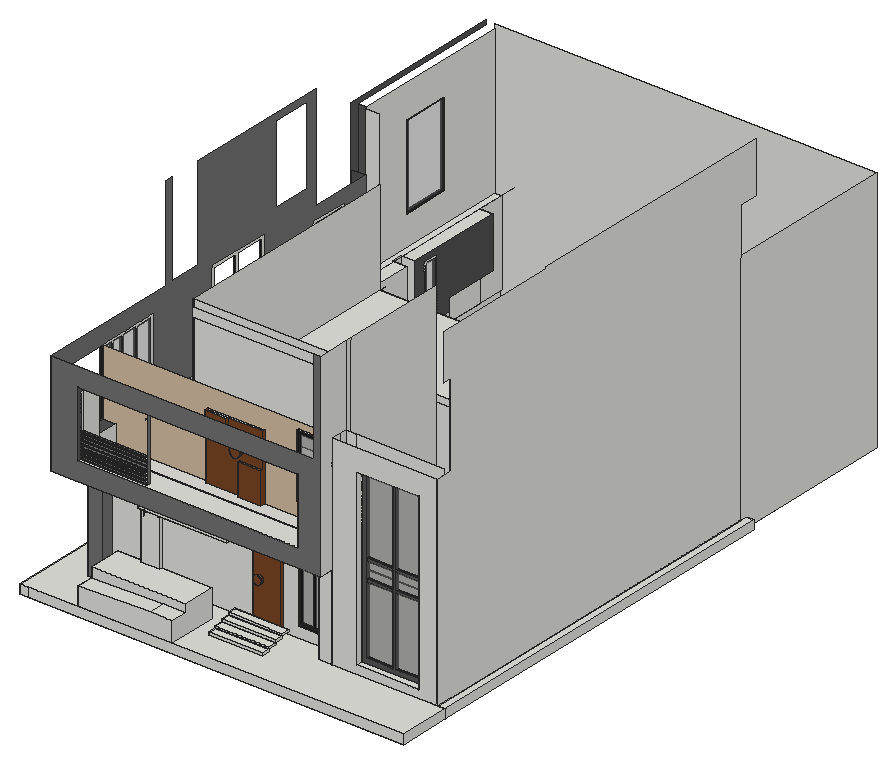
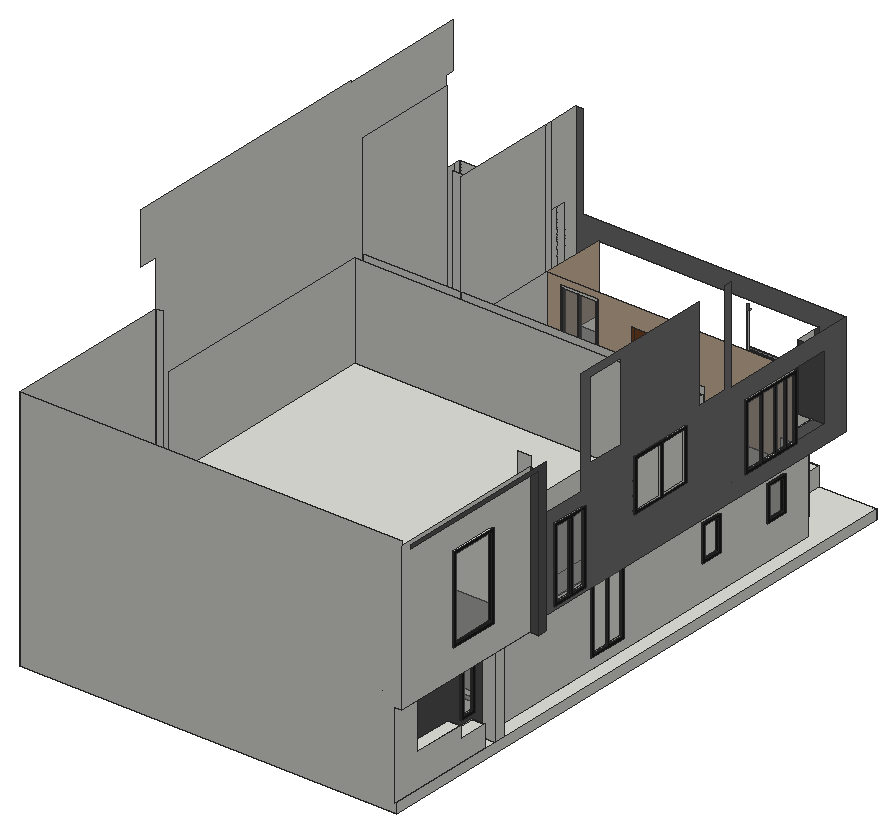
# SketchUp Ruby script. Lengths in inches.
U = 1.inch
M = Sketchup.active_model
def pt(a) = Geom::Point3d.new(a.map { |v| v * U })
def face(e, loops, mat)
  f = e.add_face(loops[0].map { |a| pt(a) })
  loops[1..].each { |l| e.add_face(l.map { |a| pt(a) }).erase! }
  f.material = f.back_material = mat if mat
  f
end
# faces: each face lists its corners as indices into pts; further lists are holes
def faces(e, pts, list, mat = nil) = list.each { |f| face(e, (f[0].is_a?(Array) ? f : [f]).map { |l| l.map { |i| pts[i] } }, mat) }
# xy, xz, yz: faces in a plane at the given z, y or x. An outline is a flat list of corners, or four numbers for a rectangle; further outlines are holes
def ring(l) = l.size == 4 ? [[l[0], l[1]], [l[2], l[1]], [l[2], l[3]], [l[0], l[3]]] : l.each_slice(2).to_a
def flat(e, list, mat, &to3) = list.each { |f| face(e, (f[0].is_a?(Array) ? f : [f]).map { |l| ring(l).map { |u, v| to3.(u, v) } }, mat) }
def xy(e, z, list, mat = nil) = flat(e, list, mat) { |x, y| [x, y, z] }
def xz(e, y, list, mat = nil) = flat(e, list, mat) { |x, z| [x, y, z] }
def yz(e, x, list, mat = nil) = flat(e, list, mat) { |y, z| [x, y, z] }
def lines(e, pts, list) = list.each { |a, b| e.add_line(pt(pts[a]), pt(pts[b])) }
# prism: a flat outline (further loops are holes) pulled along v
def prism(e, loops, v, mat = nil)
  f = face(e, loops, mat); d = Geom::Vector3d.new(v.map { |x| x * U })
  f.pushpull(f.normal.samedirection?(d) ? d.length : -d.length)
end
def box(e, o, s, mat = nil) = prism(e, [[o, [o[0] + s[0], o[1], o[2]], [o[0] + s[0], o[1] + s[1], o[2]], [o[0], o[1] + s[1], o[2]]]], [0, 0, s[2]], mat)
def at(x, y, z, deg = 0) = Geom::Transformation.translation(pt([x, y, z])) * Geom::Transformation.rotation(ORIGIN, Z_AXIS, deg.degrees)
def axes(o, x, y, z) = Geom::Transformation.new([*x, 0, *y, 0, *z, 0, *pt(o).to_a, 1])
def part(name) = M.definitions.add(name)
# library, detail: a bought-in or finely detailed component or shape, given as its bounding box
def library(name, o, s) = part(name).tap { |d| box(d.entities, o, s) }
def detail(e, o, s) = box(e.add_group.entities, o, s)
def put(e, d, t, mat = nil) = e.add_instance(d, t).tap { |i| i.material = mat if mat }
def group(e, t, mat = nil) = e.add_group.tap { |g| g.transformation = t; g.material = mat if mat }.entities
root = M.entities
M.materials.add("[0135_DarkGray]").color = [81, 81, 81]
M.materials.add("[Color M04]").color = [142, 142, 142]
M.materials.add("[Color M05]").color = [114, 114, 114]
M.materials.add("[Color M06]").color = [86, 86, 86]
M.materials.add("[Color M08]").color = [30, 30, 30]
M.materials.add("[Formica Laminate Light]").color = [213, 189, 164]
M.materials.add("[Marble Carrara Gold Floor Tile]").color = [225, 223, 217]
M.materials.add("[Translucent Glass Gray]").color = [128, 128, 128]
M.materials["[Translucent Glass Gray]"].alpha = 0.5
M.materials.add("[Wood Veneer 01]").color = [120, 70, 37]
xy(root,0,[[25.8125,0,25.8125,764.77,496.75,764.77,496.75,539.83,52.75,539.83,52.75,95.83,496.75,95.83,496.75,65.83,514.75,65.83,514.75,0],[496.75,65.83,503.64,77.83],[505.75,65.83,505.75,548.83,496.75,548.83,496.75,557.83,514.5625,557.83,514.5625,65.83],[503.64,65.83,505.75,74.83],[514.5625,65.83,514.75,557.83],
  [503.64,74.83,505.75,77.83],[503.64,74.83,505.75,86.83],[496.75,77.83,503.64,86.83],[503.64,77.83,505.75,86.83],[496.75,86.83,505.75,548.83],
  [52.75,95.83,496.75,539.83],[496.75,557.83,505.75,764.77]])
xy(root,12,[[[25.8125,0,99.13,0,99.13,63.3125,219.63,63.3125,219.63,0,514.75,0,514.75,65.83,354.09,65.83,354.09,86.83,291.2,86.83,291.2,83.83,255.2,83.83,255.2,86.83,43.75,86.83,43.75,593.74,25.8125,593.74],[68.26,54.08,88.33,68.45]],[371,65.83,496.75,65.83,496.75,548.83,43.75,548.83,43.75,86.83,371,86.83],[354.09,65.83,371,71.14],[496.75,65.83,505.75,548.83],[505.75,65.83,514.5625,557.83],
  [514.5625,65.83,514.75,557.83],[354.09,71.14,371,77.83],[354.09,77.83,371,86.83],[255.2,83.83,291.2,86.83],[496.75,548.83,505.75,557.83],
  [25.8125,607.3,43.75,607.3,43.75,622.4375,27.5,622.4375,27.5,764.77,25.8125,764.77],[27.5,622.4375,43.75,661.04],[27.5,661.04,28,730.625]])
xy(root,22.28,[[401.81,65.83,481.49,74.83],[401.81,74.83,481.49,77.83]])
xy(root,27.41,[[40.75,384.07,43.75,435.13]])
xy(root,27.74,[[313.68,83.83,351.43,86.83]])
xy(root,28.28,[[407.81,74.83,441.65,77.83],[445.14,74.83,475.49,77.83]],"[Color M06]")
xy(root,30.41,[[40.75,387.07,43.75,407.93],[40.75,409.6,43.75,432.13]],"[Color M08]")
xy(root,30.74,[[316.68,83.83,332.55,86.83],[333.49,83.83,348.43,86.83]],"[Color M08]")
xy(root,37.84,[[191.95,0,219.63,21.5625]])
xy(root,38.99,[[27.5,622.4375,43.75,661.04]])
xy(root,47.35,[[40.75,621.29,43.75,642.29]],"[Color M08]")
xy(root,48,[[99.13,21.5625,219.63,21.5625,219.63,63.3125,155.71,63.3125,155.71,59.3125,132.52,59.3125,132.52,63.3125,99.13,63.3125]])
xy(root,50.35,[[40.75,624.29,43.75,639.29]],"[Color M08]")
xy(root,54.51,[[27.5,661.04,28,730.625],[28,661.04,43.75,730.625]])
xy(root,57.8125,[[40.75,230.03,43.75,257.85]])
xy(root,57.8125,[[40.75,126.28,43.75,154.1]],"[Color M08]")
xy(root,60.8125,[[40.75,129.28,43.75,151.1],[40.75,233.03,43.75,254.85]],"[Color M08]")
xy(root,96,[[255.2,83.83,291.2,86.83]],"[Wood Veneer 01]")
xy(root,97.43,[[316.68,83.83,332.55,86.83],[333.49,83.83,348.43,86.83]],"[Color M08]")
xy(root,99.8125,[[40.75,129.28,43.75,151.1],[40.75,233.03,43.75,254.85]],"[Color M08]")
xy(root,100.43,[[313.68,83.83,351.43,86.83]],"[Color M08]")
xy(root,102.8125,[[40.75,126.28,43.75,154.1],[40.75,230.03,43.75,257.85]],"[Color M08]")
xy(root,108.125,[[132.52,59.3125,155.71,59.83],[127.97,59.83,132.52,63.3125],[155.71,59.83,155.71,63.3125,127.97,63.3125,127.97,86.83,241.41,86.83,241.41,59.83],[132.52,59.83,135.6,63.3125]])
xy(root,110.03,[[40.75,387.07,43.75,407.93],[40.75,409.6,43.75,432.13]])
xy(root,110.22,[[40.75,624.29,43.75,639.29]],"[Color M08]")
xy(root,113.03,[[40.75,384.07,43.75,435.13]],"[Color M08]")
xy(root,113.22,[[40.75,621.29,43.75,642.29]],"[Color M08]")
xy(root,115.77,[[407.81,74.83,441.65,77.83],[445.14,74.83,475.49,77.83]],"[Color M08]")
xy(root,118.37,[[407.81,74.83,441.65,77.83],[445.14,74.83,475.49,77.83]])
xy(root,120,[[354.09,65.83,371,71.14],[354.09,71.14,371,86.83],[342.51,95.83,371,230.47],[371,95.83,496.75,230.47],[51.5625,242.39,52.75,539.83],
  [52.75,242.39,496.75,539.83]])
xy(root,120,[[43.75,95.83,342.51,95.83,342.51,129.29,233.86,129.29,233.86,123.29,204.98,123.29,204.98,126.29,161.86,126.29,161.86,129.29,43.75,129.29]],"[Marble Carrara Gold Floor Tile]")
xy(root,120.1,[[19.75,548.83,19.75,764.77,27.5,764.77,27.5,730.625,43.75,730.625,43.75,607.3,25.8125,607.3,25.8125,593.74,43.75,593.74,43.75,548.83]])
xy(root,120.1,[[7.75,548.83,19.75,560.23]],"[Color M06]")
xy(root,120.125,[[27,47.14,27,548.83,43.75,548.83,43.75,86.83,127.97,86.83,127.97,59.83,241.41,59.83,241.41,86.83,371,86.83,371,47.14]])
xy(root,122.0625,[[371,85.64,496.75,86.83],[371,86.83,496.75,93.95],[371,93.95,496.75,95.83]])
xy(root,122.875,[[43.75,76.64,342.51,95.83]])
xy(root,127.17,[[24,465.2,27,514.14]],"[Color M08]")
xy(root,130.17,[[24,468.2,27,486.73],[24,489.67,27,511.14]],"[Color M08]")
xy(root,139.51,[[407.81,74.83,441.65,77.83],[445.14,74.83,475.49,77.83]],"[Color M08]")
xy(root,139.94,[[277.74,126.29,324.8,129.29]])
xy(root,140.6875,[[68.26,54.08,88.33,68.45]])
xy(root,142.35,[[407.81,74.83,441.65,77.83],[445.14,74.83,475.49,77.83]])
xy(root,142.94,[[280.74,126.29,301.27,129.29],[303.26,126.29,321.8,129.29]],"[Color M08]")
xy(root,144,[[146.02,47.14,342.51,47.14,342.51,76.64,61.54,76.64,61.54,55.45,146.02,55.45],[61.54,47.14,146.02,53.64],[61.54,53.64,145.89,55.45],[145.89,53.64,146.02,55.45],[43.75,76.64,61.54,80.27]])
xy(root,144,[[27,80.27,43.75,129.29]],"[0135_DarkGray]")
xy(root,144,[[24,129.29,27,209.85]],"[Color M08]")
xy(root,145.3125,[[61.54,49.95,146.02,53.64]])
xy(root,146.39,[[61.54,49.95,146.02,53.64]],"[Color M05]")
xy(root,147,[[24,132.29,27,144.3],[24,146.33,27,160.37],[24,161.62,27,182.61],[24,184.3,27,206.85]])
xy(root,149.6875,[[61.54,49.95,146.02,53.64]],"[Color M05]")
xy(root,150.77,[[61.54,49.95,146.02,53.64]],"[Color M05]")
xy(root,154.0625,[[61.54,49.95,146.02,53.64]],"[Color M05]")
xy(root,155.14,[[61.54,49.95,146.02,53.64]],"[Color M05]")
xy(root,157.5,[[16.75,621.57,19.75,684.82]],"[Color M08]")
xy(root,158.4375,[[61.54,49.95,146.02,53.64]],"[Color M05]")
xy(root,159.52,[[61.54,49.95,146.02,53.64]],"[Color M05]")
xy(root,160.11,[[204.98,123.29,233.86,126.29]],"[Wood Veneer 01]")
xy(root,160.5,[[16.75,624.57,19.75,681.82]],"[Color M08]")
xy(root,162.8125,[[61.54,49.95,146.02,53.64]],"[Color M05]")
xy(root,163.89,[[61.54,49.95,146.02,53.64]],"[Color M05]")
xy(root,167.1875,[[61.54,49.95,146.02,53.64]],"[Color M05]")
xy(root,168.27,[[61.54,49.95,146.02,53.64]],"[Color M05]")
xy(root,171.5625,[[61.54,49.95,146.02,53.64]],"[Color M05]")
xy(root,172.64,[[61.54,49.95,146.02,53.64]],"[Color M05]")
xy(root,175.66,[[24,303.96,27,386.64]],"[Color M08]")
xy(root,175.9375,[[61.54,49.95,146.02,53.64]],"[Color M05]")
xy(root,176.1875,[[161.86,123.29,189.67,126.29]],"[Wood Veneer 01]")
xy(root,177.02,[[61.54,49.95,146.02,53.64]],"[Color M05]")
xz(root,0,[[25.8125,0,34.75,12],[34.75,0,514.75,12],[99.13,12,219.63,12,219.63,37.84,191.95,37.84,99.13,35.36]])
xz(root,21.5625,[[99.13,35.36,191.95,37.84,219.63,37.84,219.63,48,99.13,48]])
xz(root,47.14,[[[27,120.125,371,120.125,371,372,362,372,362,252,27,252],[61.54,144,342.51,228.48]]],"[Color M05]")
xz(root,49.95,[[61.54,154.0625,146.02,155.14]],"[Color M04]")
xz(root,49.95,[[61.54,145.3125,146.02,146.39],[61.54,149.6875,146.02,150.77],[61.54,158.4375,146.02,159.52],[61.54,162.8125,146.02,163.89],[61.54,167.1875,146.02,168.27],
  [61.54,171.5625,146.02,172.64],[61.54,175.9375,146.02,177.02]],"[Color M05]")
xz(root,53.64,[[61.54,137.64,146.02,140.9375],[61.54,142.02,146.02,144],[145.89,144,146.02,145.3125],[61.54,145.3125,145.89,146.39],[145.89,145.3125,146.02,146.39],
  [145.89,146.39,146.02,149.6875],[61.54,149.6875,145.89,150.77],[145.89,149.6875,146.02,150.77],[145.89,150.77,146.02,154.0625],[61.54,154.0625,145.89,155.14],
  [145.89,154.0625,146.02,155.14],[145.89,155.14,146.02,158.4375],[61.54,158.4375,145.89,159.52],[145.89,158.4375,146.02,159.52],[145.89,159.52,146.02,162.8125],
  [61.54,162.8125,145.89,163.89],[145.89,162.8125,146.02,163.89],[145.89,163.89,146.02,167.1875],[61.54,167.1875,145.89,168.27],[145.89,167.1875,146.02,168.27],
  [145.89,168.27,146.02,171.5625],[61.54,171.5625,145.89,172.64],[145.89,171.5625,146.02,172.64],[145.89,172.64,146.02,175.9375],[61.54,175.9375,145.89,177.02],
  [145.89,175.9375,146.02,177.02],[145.89,177.02,146.02,180.3125]])
xz(root,54.08,[[68.26,12,88.33,140.6875]],"[Color M05]")
xz(root,55.45,[[145.89,144,146.02,220.77]])
xz(root,59.3125,[[132.52,48,155.71,108.125]])
xz(root,59.83,[[127.97,108.125,241.41,120.125]])
xz(root,63.3125,[[99.13,12,99.13,48,132.52,48,132.52,108.125,135.6,108.125,135.6,101.9375,155.71,101.9375,155.71,48,219.63,48,219.63,12],[135.6,101.9375,155.71,108.125]])
xz(root,65.83,[[496.75,0,503.64,12],[503.64,0,505.75,12],[505.75,0,514.5625,12],[514.5625,0,514.75,12],[354.09,12,371,120],
  [[371,12,503.64,270.8125],[401.81,22.28,481.49,243.28]],[503.64,12,505.75,270.8125]])
xz(root,68.45,[[68.26,12,88.33,140.6875]])
xz(root,71.14,[[354.09,12,371,120]])
xz(root,74.83,[[[401.81,22.28,481.49,243.28],[407.81,28.28,407.81,237.28,441.65,237.28,441.65,142.35,407.81,142.35,407.81,139.51,441.65,139.51,441.65,118.37,407.81,118.37,407.81,115.77,441.65,115.77,441.65,28.28],[445.14,142.35,475.49,237.28],[445.14,28.28,475.49,115.77],[445.14,118.37,475.49,139.51]]],"[Color M06]")
xz(root,76.64,[[43.75,122.875,342.51,144]])
xz(root,77.83,[[[401.81,22.28,481.49,243.28],[407.81,28.28,441.65,28.28,441.65,115.77,407.81,115.77,407.81,118.37,441.65,118.37,441.65,139.51,407.81,139.51,407.81,142.35,441.65,142.35,441.65,237.28,407.81,237.28],[445.14,142.35,475.49,237.28],[445.14,28.28,475.49,115.77],[445.14,118.37,475.49,139.51]]])
xz(root,77.83,[[407.81,28.28,441.65,115.77],[445.14,28.28,475.49,115.77],[407.81,118.37,441.65,139.51],[445.14,118.37,475.49,139.51],[407.81,142.35,441.65,237.28],
  [445.14,142.35,475.49,237.28]],"[Translucent Glass Gray]")
xz(root,80.27,[[27,144,61.54,228.4375]],"[0135_DarkGray]")
xz(root,80.83,[[263.32,58.23,264.76,58.52,266.08,59.16,267.18,60.125,268,61.34,268.48,62.73,268.58,64.19,268.3,65.64,267.66,66.96,266.7,68.0625,265.48,68.88,264.09,69.36,262.625,69.46,261.18,69.18,259.86,68.54,258.76,67.58,257.94,66.36,257.46,64.97,257.36,63.5,257.64,62.0625,258.28,60.74,259.24,59.64,260.46,58.81,261.85,58.34]],"[Wood Veneer 01]")
xz(root,83.83,[[[313.68,27.74,351.43,100.43],[316.68,30.74,332.55,97.43],[333.49,30.74,348.43,97.43]]],"[Color M08]")
xz(root,83.83,[[[255.2,12,291.2,96],[263.32,58.23,261.85,58.34,260.46,58.81,259.24,59.64,258.28,60.74,257.64,62.0625,257.36,63.5,257.46,64.97,257.94,66.36,258.76,67.58,259.86,68.54,261.18,69.18,262.625,69.46,264.09,69.36,265.48,68.88,266.7,68.0625,267.66,66.96,268.3,65.64,268.58,64.19,268.48,62.73,268,61.34,267.18,60.125,266.08,59.16,264.76,58.52]]],"[Wood Veneer 01]")
xz(root,86.83,[[[43.75,12,255.2,12,255.2,96,291.2,96,291.2,12,354.09,12,354.09,120,371,120,371,120.125,241.41,120.125,241.41,108.125,127.97,108.125,127.97,120.125,43.75,120.125],[313.68,27.74,351.43,100.43]],[255.2,12,291.2,96],[[313.68,27.74,351.43,100.43],[316.68,30.74,332.55,97.43],[333.49,30.74,348.43,97.43]],[371,120,383.7,122.0625],[371,122.0625,383.7,270.8125],
  [383.7,122.0625,496.75,270.8125]])
xz(root,86.83,[[316.68,30.74,332.55,97.43],[333.49,30.74,348.43,97.43]],"[Translucent Glass Gray]")
xz(root,95.83,[[52.75,0,496.75,120],[43.75,120,342.51,122.875],[371,120,496.75,122.0625]])
xz(root,123.29,[[204.98,120,233.86,160.11],[200.35,162.67,202.08,162.9,203.69,163.5625,205.08,164.625,206.14,166.01,206.8125,167.625,207.04,169.36,206.8125,171.09,206.14,172.7,205.08,174.08,203.69,175.15,202.08,175.81,200.35,176.04,198.62,175.81,197.01,175.15,195.62,174.08,194.56,172.7,193.89,171.09,193.66,169.36,193.89,167.625,194.56,166.01,195.62,164.625,197.01,163.5625,198.62,162.9],[161.86,176.1875,189.67,204]],"[Wood Veneer 01]")
xz(root,126.28,[[40.75,57.8125,43.75,102.8125]],"[Color M08]")
xz(root,126.29,[[[277.74,139.94,324.8,220.37],[280.74,142.94,280.74,217.37,321.8,217.37,321.8,142.94,303.26,142.94,303.26,217.37,301.27,217.37,301.27,142.94]]],"[Color M08]")
xz(root,126.29,[[[161.86,120,204.98,120,204.98,160.11,233.86,160.11,233.86,204,189.67,204,189.67,176.1875,161.86,176.1875],[200.35,162.67,198.62,162.9,197.01,163.5625,195.62,164.625,194.56,166.01,193.89,167.625,193.66,169.36,193.89,171.09,194.56,172.7,195.62,174.08,197.01,175.15,198.62,175.81,200.35,176.04,202.08,175.81,203.69,175.15,205.08,174.08,206.14,172.7,206.8125,171.09,207.04,169.36,206.8125,167.625,206.14,166.01,205.08,164.625,203.69,163.5625,202.08,162.9]]],"[Wood Veneer 01]")
xz(root,129.28,[[40.75,60.8125,43.75,99.8125]],"[Color M08]")
xz(root,129.29,[[[277.74,139.94,324.8,220.37],[280.74,142.94,301.27,142.94,301.27,217.37,303.26,217.37,303.26,142.94,321.8,142.94,321.8,217.37,280.74,217.37]]])
xz(root,129.29,[[24,144,27,228.48]],"[Color M08]")
xz(root,129.29,[[[43.75,120,161.86,120,161.86,204,233.86,204,233.86,120,342.51,120,342.51,228.48,27,228.48,27,144,43.75,144],[277.74,139.94,324.8,220.37]]],"[Formica Laminate Light]")
xz(root,129.29,[[280.74,142.94,301.27,217.37],[303.26,142.94,321.8,217.37]],"[Translucent Glass Gray]")
xz(root,132.29,[[24,147,27,225.48]],"[Color M08]")
xz(root,144.3,[[24,147,27,225.48]],"[Color M08]")
xz(root,146.33,[[24,147,27,225.48]],"[Color M08]")
xz(root,151.1,[[40.75,60.8125,43.75,99.8125]],"[Color M08]")
xz(root,154.1,[[40.75,57.8125,43.75,102.8125]],"[Color M08]")
xz(root,160.37,[[24,147,27,225.48]],"[Color M08]")
xz(root,161.62,[[24,147,27,225.48]],"[Color M08]")
xz(root,182.61,[[24,147,27,225.48]],"[Color M08]")
xz(root,184.3,[[24,147,27,225.48]],"[Color M08]")
xz(root,206.85,[[24,147,27,225.48]],"[Color M08]")
xz(root,209.85,[[24,144,27,228.48]],"[Color M08]")
xz(root,230.03,[[40.75,57.8125,43.75,102.8125]],"[Color M08]")
xz(root,230.47,[[43.75,120,52.75,120.125],[342.51,120,371,120,371,240,61.54,240,61.54,228.48,342.51,228.48],[371,120,496.75,240],[43.75,120.125,52.75,144]])
xz(root,233.03,[[40.75,60.8125,43.75,99.8125]],"[Color M08]")
xz(root,242.39,[[51.5625,120,52.75,240],[52.75,120,496.75,240]])
xz(root,254.85,[[40.75,60.8125,43.75,99.8125]],"[Color M08]")
xz(root,257.85,[[40.75,57.8125,43.75,102.8125]],"[Color M08]")
xz(root,303.96,[[24,175.66,27,241.72]],"[Color M08]")
xz(root,384.07,[[40.75,27.41,43.75,113.03]],"[Color M08]")
xz(root,386.64,[[24,175.66,27,241.72]],"[Color M08]")
xz(root,387.07,[[40.75,30.41,43.75,110.03]],"[Color M08]")
xz(root,407.93,[[40.75,30.41,43.75,110.03]],"[Color M08]")
xz(root,409.6,[[40.75,30.41,43.75,110.03]],"[Color M08]")
xz(root,432.13,[[40.75,30.41,43.75,110.03]],"[Color M08]")
xz(root,435.13,[[40.75,27.41,43.75,113.03]],"[Color M08]")
xz(root,465.2,[[24,127.17,27,221.17]],"[Color M08]")
xz(root,468.2,[[24,130.17,27,218.17]],"[Color M08]")
xz(root,486.73,[[24,130.17,27,218.17]],"[Color M08]")
xz(root,489.67,[[24,130.17,27,218.17]],"[Color M08]")
xz(root,511.14,[[24,130.17,27,218.17]],"[Color M08]")
xz(root,514.14,[[24,127.17,27,221.17]],"[Color M08]")
xz(root,539.83,[[52.75,0,496.75,120],[51.5625,120,52.75,240]])
xz(root,548.83,[[496.75,12,505.75,313.6875],[27,120.1,43.75,120.125],[27,120.125,43.75,144],[27,144,43.75,313.6875]])
xz(root,548.83,[[7.75,120.1,27,238.0625]],"[0135_DarkGray]")
xz(root,557.83,[[496.75,0,505.75,12],[505.75,0,514.3125,12],[514.3125,0,514.5625,12],[514.5625,0,514.75,12]])
xz(root,560.23,[[7.75,120.1,19.75,308.3]],"[Color M06]")
xz(root,593.74,[[25.8125,12,43.75,120.1]])
xz(root,607.3,[[25.8125,12,43.75,120.1]])
xz(root,621.29,[[40.75,47.35,43.75,113.22]],"[Color M08]")
xz(root,621.57,[[16.75,157.5,19.75,266.93]],"[Color M08]")
xz(root,622.4375,[[27.5,12,43.75,38.99]])
xz(root,624.29,[[40.75,50.35,43.75,110.22]],"[Color M08]")
xz(root,624.57,[[16.75,160.5,19.75,263.93]],"[Color M08]")
xz(root,639.29,[[40.75,50.35,43.75,110.22]],"[Color M08]")
xz(root,642.29,[[40.75,47.35,43.75,113.22]],"[Color M08]")
xz(root,661.04,[[27.5,38.99,43.75,54.51]])
xz(root,681.82,[[16.75,160.5,19.75,263.93]],"[Color M08]")
xz(root,684.82,[[16.75,157.5,19.75,266.93]],"[Color M08]")
xz(root,730.625,[[27.5,54.51,43.75,120.1]])
xz(root,764.77,[[25.8125,0,25.8125,12,27.5,12,27.5,120.1,19.75,120.1,19.75,313.6875,505.75,313.6875,505.75,0]])
yz(root,7.75,[[548.83,120.1,548.83,313.6875,764.77,313.6875,764.77,308.3,560.23,308.3,560.23,120.1]],"[Color M06]")
yz(root,16.75,[[[621.57,157.5,684.82,266.93],[624.57,160.5,681.82,263.93]]],"[Color M08]")
yz(root,19.75,[[[560.23,120.1,764.77,308.3],[621.57,157.5,684.82,266.93]]])
yz(root,19.75,[[624.57,160.5,681.82,263.93]],"[Translucent Glass Gray]")
yz(root,24,[[[465.2,127.17,514.14,221.17],[489.67,130.17,511.14,218.17],[468.2,130.17,486.73,218.17]],[[129.29,144,209.85,228.48],[184.3,147,206.85,225.48],[161.62,147,182.61,225.48],[146.33,147,160.37,225.48],[132.29,147,144.3,225.48]],[[303.96,175.66,386.64,241.72],[345.3,178.66,383.64,238.72],[306.96,178.66,342.36,238.72]]],"[Color M08]")
yz(root,25.8125,[[0,0,764.77,12],[593.74,12,607.3,120.1]])
yz(root,27,[[[465.2,127.17,514.14,221.17],[489.67,130.17,511.14,218.17],[468.2,130.17,486.73,218.17]],[[129.29,144,209.85,228.48],[184.3,147,206.85,225.48],[161.62,147,182.61,225.48],[146.33,147,160.37,225.48],[132.29,147,144.3,225.48]],[[303.96,175.66,386.64,241.72],[345.3,178.66,383.64,238.72],[306.96,178.66,342.36,238.72]]])
yz(root,27,[[[47.14,120.125,47.14,252,230.47,252,230.47,372,239.47,372,239.47,252.8125,281.29,252.8125,281.29,372,469.72,372,469.72,238.0625,548.83,238.0625,548.83,120.125],[80.27,144,209.85,228.48],[303.96,175.66,386.64,241.72],[405.68,263.61,454.62,362.86],[465.2,127.17,514.14,221.17]]],"[Color M05]")
yz(root,27,[[468.2,130.17,486.73,218.17],[489.67,130.17,511.14,218.17],[132.29,147,144.3,225.48],[146.33,147,160.37,225.48],[161.62,147,182.61,225.48],
  [184.3,147,206.85,225.48]],"[Translucent Glass Gray]")
yz(root,27.5,[[622.4375,12,622.4375,38.99,661.04,38.99,661.04,54.51,730.625,54.51,730.625,120.1,764.77,120.1,764.77,12]])
yz(root,40.75,[[[384.07,27.41,435.13,113.03],[409.6,30.41,432.13,110.03],[387.07,30.41,407.93,110.03]],[[621.29,47.35,642.29,113.22],[624.29,50.35,639.29,110.22]],[[126.28,57.8125,154.1,102.8125],[129.28,60.8125,151.1,99.8125]],[[230.03,57.8125,257.85,102.8125],[233.03,60.8125,254.85,99.8125]]],"[Color M08]")
yz(root,43.75,[[[86.83,12,86.83,120,548.83,120,548.83,120.1,593.74,120.1,593.74,12],[384.07,27.41,435.13,113.03],[230.03,57.8125,257.85,102.8125],[126.28,57.8125,154.1,102.8125]],[622.4375,12,661.04,38.99],[[384.07,27.41,435.13,113.03],[409.6,30.41,432.13,110.03],[387.07,30.41,407.93,110.03]],[[621.29,47.35,642.29,113.22],[624.29,50.35,639.29,110.22]],[86.83,120,95.83,120.125],
  [95.83,120,129.29,120.125],[129.29,120,230.47,120.125],[230.47,120,548.83,120.125],[95.83,120.125,129.29,120.125,129.29,144,76.64,144,76.64,122.875,95.83,122.875],[230.47,120.125,548.83,144]])
yz(root,43.75,[[[607.3,12,607.3,120.1,730.625,120.1,730.625,54.51,661.04,54.51,661.04,38.99,622.4375,38.99,622.4375,12],[621.29,47.35,642.29,113.22]]],"[0135_DarkGray]")
yz(root,43.75,[[387.07,30.41,407.93,110.03],[409.6,30.41,432.13,110.03],[624.29,50.35,639.29,110.22],[129.28,60.8125,151.1,99.8125],[233.03,60.8125,254.85,99.8125]],"[Translucent Glass Gray]")
yz(root,52.75,[[242.39,120,539.83,240]])
yz(root,61.54,[[53.64,144,55.45,144,55.45,220.77,50.64,220.77,50.64,219.6875,53.64,219.6875],[55.45,144,80.27,228.4375],[49.95,145.3125,53.64,146.39],[49.95,149.6875,53.64,150.77],[49.95,154.0625,53.64,155.14],
  [49.95,158.4375,53.64,159.52],[49.95,162.8125,53.64,163.89],[49.95,167.1875,53.64,168.27],[49.95,171.5625,53.64,172.64],[49.95,175.9375,53.64,177.02]])
yz(root,61.54,[[47.14,144,53.64,144,53.64,145.3125,49.95,145.3125,49.95,146.39,53.64,146.39,53.64,149.6875,49.95,149.6875,49.95,150.77,53.64,150.77,53.64,154.0625,49.95,154.0625,49.95,155.14,53.64,155.14,53.64,158.4375,49.95,158.4375,49.95,159.52,53.64,159.52,53.64,162.8125,49.95,162.8125,49.95,163.89,53.64,163.89,53.64,167.1875,49.95,167.1875,49.95,168.27,53.64,168.27,53.64,171.5625,49.95,171.5625,49.95,172.64,53.64,172.64,53.64,175.9375,49.95,175.9375,49.95,177.02,53.64,177.02,53.64,180.3125,49.95,180.3125,49.95,181.39,53.64,181.39,53.64,184.6875,49.95,184.6875,49.95,185.77,53.64,185.77,53.64,189.0625,49.95,189.0625,49.95,190.14,53.64,190.14,53.64,193.4375,49.95,193.4375,49.95,194.52,53.64,194.52,53.64,197.8125,49.95,197.8125,49.95,198.89,53.64,198.89,53.64,202.1875,49.95,202.1875,49.95,203.27,53.64,203.27,53.64,206.5625,49.95,206.5625,49.95,207.64,53.64,207.64,53.64,210.9375,50.64,210.9375,50.64,212.02,53.64,212.02,53.64,215.3125,50.64,215.3125,50.64,216.39,53.64,216.39,53.64,219.6875,50.64,219.6875,50.64,220.77,55.45,220.77,55.45,224.0625,53.64,224.0625,53.64,228.4375,47.14,228.4375]],"[Color M06]")
yz(root,68.26,[[54.08,12,68.45,140.6875]],"[Color M05]")
yz(root,88.33,[[54.08,12,68.45,140.6875]],"[Color M05]")
yz(root,99.13,[[0,12,0,35.36,21.5625,35.36,21.5625,48,63.3125,48,63.3125,12]])
yz(root,127.97,[[59.83,108.125,86.83,120.125]])
yz(root,132.52,[[59.3125,48,63.3125,108.125]])
yz(root,135.6,[[59.83,101.9375,63.3125,108.125]])
yz(root,145.89,[[53.64,144,53.64,219.6875,50.64,219.6875,50.64,220.77,55.45,220.77,55.45,144]])
yz(root,146.02,[[53.64,144,55.45,228.48],[49.95,145.3125,53.64,146.39],[49.95,149.6875,53.64,150.77],[49.95,154.0625,53.64,155.14],[49.95,158.4375,53.64,159.52],
  [49.95,162.8125,53.64,163.89],[49.95,167.1875,53.64,168.27],[49.95,171.5625,53.64,172.64],[49.95,175.9375,53.64,177.02]],"[Color M05]")
yz(root,155.71,[[59.3125,48,63.3125,108.125]])
yz(root,161.86,[[126.29,120,126.29,176.1875,123.29,176.1875,123.29,204,129.29,204,129.29,120]],"[Wood Veneer 01]")
yz(root,189.67,[[123.29,176.1875,126.29,204]],"[Wood Veneer 01]")
yz(root,204.98,[[123.29,120,126.29,160.11]],"[Wood Veneer 01]")
yz(root,219.63,[[0,12,63.3125,12,63.3125,48,21.5625,48,21.5625,37.84,0,37.84]])
yz(root,233.86,[[123.29,120,129.29,120,129.29,204,126.29,204,126.29,160.11,123.29,160.11]],"[Wood Veneer 01]")
yz(root,241.41,[[59.83,108.125,86.83,120.125]])
yz(root,255.2,[[83.83,12,86.83,96]],"[Wood Veneer 01]")
yz(root,277.74,[[126.29,139.94,129.29,220.37]],"[Color M08]")
yz(root,280.74,[[126.29,142.94,129.29,217.37]],"[Color M08]")
yz(root,291.2,[[83.83,12,86.83,96]],"[Wood Veneer 01]")
yz(root,301.27,[[126.29,142.94,129.29,217.37]],"[Color M08]")
yz(root,303.26,[[126.29,142.94,129.29,217.37]],"[Color M08]")
yz(root,313.68,[[83.83,27.74,86.83,100.43]],"[Color M08]")
yz(root,316.68,[[83.83,30.74,86.83,97.43]],"[Color M08]")
yz(root,321.8,[[126.29,142.94,129.29,217.37]],"[Color M08]")
yz(root,324.8,[[126.29,139.94,129.29,220.37]],"[Color M08]")
yz(root,332.55,[[83.83,30.74,86.83,97.43]],"[Color M08]")
yz(root,333.49,[[83.83,30.74,86.83,97.43]],"[Color M08]")
yz(root,342.51,[[129.29,120,230.47,228.48]])
yz(root,342.51,[[95.83,120,95.83,122.875,76.64,122.875,76.64,144,47.14,144,47.14,228.48,129.29,228.48,129.29,120]],"[Formica Laminate Light]")
yz(root,348.43,[[83.83,30.74,86.83,97.43]],"[Color M08]")
yz(root,351.43,[[83.83,27.74,86.83,100.43]])
yz(root,354.09,[[65.83,12,71.14,120],[71.14,12,86.83,120]])
yz(root,371,[[65.83,12,71.14,120],[71.14,12,86.83,120],[65.83,120,77.83,120.125],[77.83,120,85.64,120.125],[85.64,120,86.83,120.125],
  [86.83,120,93.95,120.125],[95.83,120,230.47,372],[47.14,120.125,65.83,120.125,65.83,270.8125,86.83,270.8125,86.83,372,47.14,372],[65.83,120.125,77.83,270.8125],[77.83,120.125,85.64,120.125,85.64,122.0625,86.83,122.0625,86.83,270.8125,77.83,270.8125],
  [85.64,120.125,86.83,122.0625],[86.83,120.125,93.95,122.0625],[86.83,122.0625,95.83,372]])
yz(root,401.81,[[65.83,22.28,74.83,243.28],[74.83,22.28,77.83,243.28]])
yz(root,407.81,[[74.83,115.77,77.83,118.37],[74.83,139.51,77.83,142.35]])
yz(root,407.81,[[74.83,28.28,77.83,115.77],[74.83,118.37,77.83,139.51],[74.83,142.35,77.83,237.28]],"[Color M06]")
yz(root,441.65,[[74.83,28.28,77.83,115.77],[74.83,118.37,77.83,139.51],[74.83,142.35,77.83,237.28]],"[Color M06]")
yz(root,445.14,[[74.83,28.28,77.83,115.77],[74.83,118.37,77.83,139.51],[74.83,142.35,77.83,237.28]],"[Color M06]")
yz(root,475.49,[[74.83,28.28,77.83,115.77],[74.83,118.37,77.83,139.51],[74.83,142.35,77.83,237.28]],"[Color M06]")
yz(root,481.49,[[65.83,22.28,74.83,243.28],[74.83,22.28,77.83,243.28]])
yz(root,496.75,[[65.83,0,95.83,12],[95.83,0,539.83,12],[539.83,0,557.83,12],[95.83,120,230.47,122.0625],[242.39,120,539.83,240],
  [95.83,122.0625,230.47,372]])
yz(root,505.75,[[65.83,0,86.83,12],[86.83,0,548.83,12],[557.83,0,764.77,0,764.77,313.6875,548.83,313.6875,548.83,12,557.83,12],[65.83,12,548.83,12,548.83,372,572.83,372,572.83,437.4375,238.52,437.4375,238.52,435.13,74.83,435.13,74.83,377.09,86.83,377.09,86.83,270.8125,65.83,270.8125]])
yz(root,514.5625,[[65.83,0,557.83,12]])
yz(root,514.75,[[0,0,65.83,12]])
p = [[191.95,21.5625,37.84],[99.13,21.5625,35.36],[99.13,0,35.36],[191.95,0,37.84],[261.85,83.83,58.34],[263.32,83.83,58.23],
  [263.32,80.83,58.23],[261.85,80.83,58.34],[264.76,83.83,58.52],[264.76,80.83,58.52],[260.46,83.83,58.81],[260.46,80.83,58.81],
  [266.08,83.83,59.16],[266.08,80.83,59.16],[259.24,83.83,59.64],[259.24,80.83,59.64],[267.18,83.83,60.125],[267.18,80.83,60.125],
  [258.28,83.83,60.74],[258.28,80.83,60.74],[268,83.83,61.34],[268,80.83,61.34],[257.64,83.83,62.0625],[257.64,80.83,62.0625],
  [268.48,83.83,62.73],[268.48,80.83,62.73],[257.36,83.83,63.5],[257.36,80.83,63.5],[268.58,83.83,64.19],[268.58,80.83,64.19],
  [257.46,83.83,64.97],[257.46,80.83,64.97],[268.3,83.83,65.64],[268.3,80.83,65.64],[257.94,83.83,66.36],[257.94,80.83,66.36],
  [267.66,83.83,66.96],[267.66,80.83,66.96],[258.76,83.83,67.58],[258.76,80.83,67.58],[266.7,83.83,68.0625],[266.7,80.83,68.0625],
  [259.86,83.83,68.54],[259.86,80.83,68.54],[265.48,83.83,68.88],[265.48,80.83,68.88],[261.18,83.83,69.18],[261.18,80.83,69.18],
  [264.09,83.83,69.36],[264.09,80.83,69.36],[262.625,83.83,69.46],[262.625,80.83,69.46],[198.62,126.29,162.9],[200.35,126.29,162.67],
  [200.35,123.29,162.67],[198.62,123.29,162.9],[202.08,126.29,162.9],[202.08,123.29,162.9],[197.01,126.29,163.5625],[197.01,123.29,163.5625],
  [203.69,126.29,163.5625],[203.69,123.29,163.5625],[195.62,126.29,164.625],[195.62,123.29,164.625],[205.08,126.29,164.625],[205.08,123.29,164.625],
  [194.56,126.29,166.01],[194.56,123.29,166.01],[206.14,126.29,166.01],[206.14,123.29,166.01],[193.89,126.29,167.625],[193.89,123.29,167.625],
  [206.8125,126.29,167.625],[206.8125,123.29,167.625],[193.66,126.29,169.36],[193.66,123.29,169.36],[207.04,126.29,169.36],[207.04,123.29,169.36],
  [193.89,126.29,171.09],[193.89,123.29,171.09],[206.8125,126.29,171.09],[206.8125,123.29,171.09],[194.56,126.29,172.7],[194.56,123.29,172.7],
  [206.14,126.29,172.7],[206.14,123.29,172.7],[195.62,126.29,174.08],[195.62,123.29,174.08],[205.08,126.29,174.08],[205.08,123.29,174.08],
  [197.01,126.29,175.15],[197.01,123.29,175.15],[203.69,126.29,175.15],[203.69,123.29,175.15],[198.62,126.29,175.81],[198.62,123.29,175.81],
  [202.08,126.29,175.81],[202.08,123.29,175.81],[200.35,126.29,176.04],[200.35,123.29,176.04],[43.75,86.83,0],[43.75,86.83,12],
  [43.75,548.83,0],[43.75,548.83,12],[52.75,230.47,120],[52.75,129.29,120],[52.75,242.39,120],[52.75,548.83,120],
  [52.75,539.83,120],[52.75,230.47,144],[52.75,174.66,144],[43.75,230.47,144],[27,230.47,144],[503.64,74.83,270.8125],
  [503.64,74.83,0],[383.7,86.83,120],[383.7,86.83,0],[503.64,86.83,120],[503.64,77.83,120],[371,86.83,12],
  [371,86.83,0],[135.6,59.83,101.9375],[155.71,59.83,101.9375],[371,65.83,0],[371,65.83,12],[383.7,65.83,0],
  [383.7,65.83,12],[43.75,764.77,134.95],[43.75,550.11,134.95],[28,730.625,12],[28,730.625,54.51]]
faces(root,p,[[0,1,2,3]])
faces(root,p,[[4,5,6,7],[5,8,9,6],[10,4,7,11],[8,12,13,9],[14,10,11,15],[12,16,17,13],[18,14,15,19],[16,20,21,17],
  [22,18,19,23],[20,24,25,21],[26,22,23,27],[24,28,29,25],[30,26,27,31],[28,32,33,29],[34,30,31,35],[32,36,37,33],
  [38,34,35,39],[36,40,41,37],[42,38,39,43],[40,44,45,41],[46,42,43,47],[44,48,49,45],[50,46,47,51],[48,50,51,49],
  [52,53,54,55],[53,56,57,54],[58,52,55,59],[56,60,61,57],[62,58,59,63],[60,64,65,61],[66,62,63,67],[64,68,69,65],
  [70,66,67,71],[68,72,73,69],[74,70,71,75],[72,76,77,73],[78,74,75,79],[76,80,81,77],[82,78,79,83],[80,84,85,81],
  [86,82,83,87],[84,88,89,85],[90,86,87,91],[88,92,93,89],[94,90,91,95],[92,96,97,93],[98,94,95,99],[96,98,99,97]],"[Wood Veneer 01]")
lines(root,p,[[100,101],[102,103],[104,105],[106,104],[107,108],[109,110],[111,112],[113,114],[115,116],[117,118],[119,120],[121,122],
  [123,124],[125,126],[127,128],[129,130]])
g1 = group(root,at(237.27,36.08,12))
xy(g1,0,[[0,0,68.6875,10.4375]])
xy(g1,3,[[0,0,68.6875,10.4375],[0,10.4375,68.6875,20.875]])
xy(g1,6,[[0,10.4375,68.6875,20.875],[0,20.875,68.6875,31.3125]])
xy(g1,9,[[0,20.875,68.6875,31.3125],[0,31.3125,68.6875,41.75]])
xy(g1,12,[[0,31.3125,68.6875,41.75]])
xz(g1,0,[[0,0,68.6875,3]])
xz(g1,10.4375,[[0,0,68.6875,3],[0,3,68.6875,6]])
xz(g1,20.875,[[0,3,68.6875,6],[0,6,68.6875,9]])
xz(g1,31.3125,[[0,6,68.6875,9],[0,9,68.6875,12]])
xz(g1,41.75,[[0,9,68.6875,12]])
yz(g1,0,[[0,0,10.4375,3],[10.4375,3,20.875,6],[20.875,6,31.3125,9],[31.3125,9,41.75,12]])
yz(g1,68.6875,[[0,0,10.4375,3],[10.4375,3,20.875,6],[20.875,6,31.3125,9],[31.3125,9,41.75,12]])
